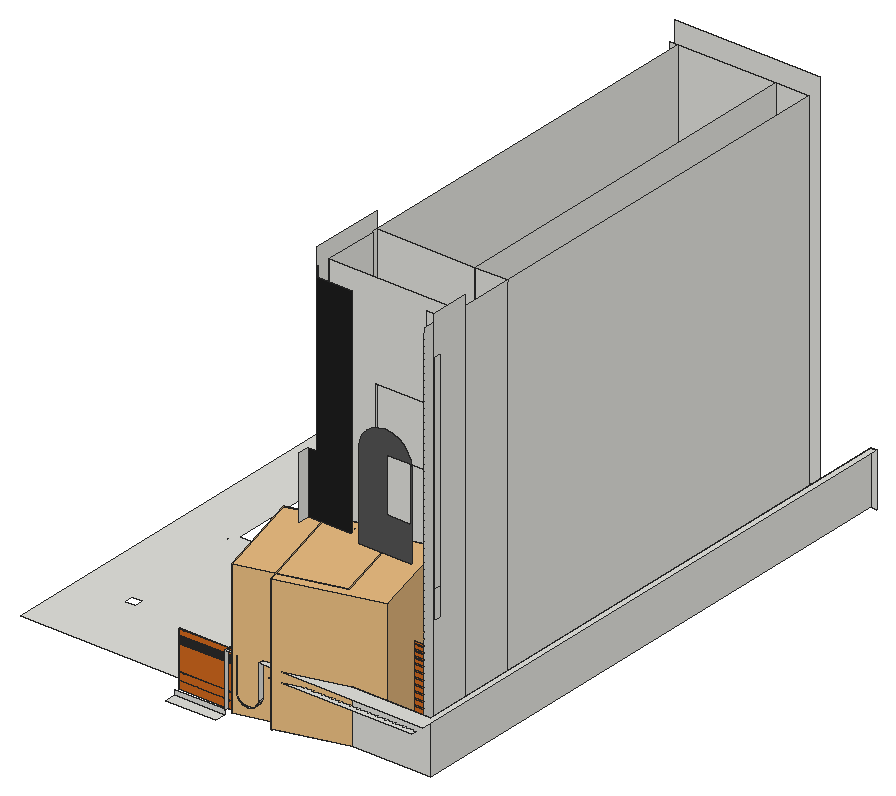
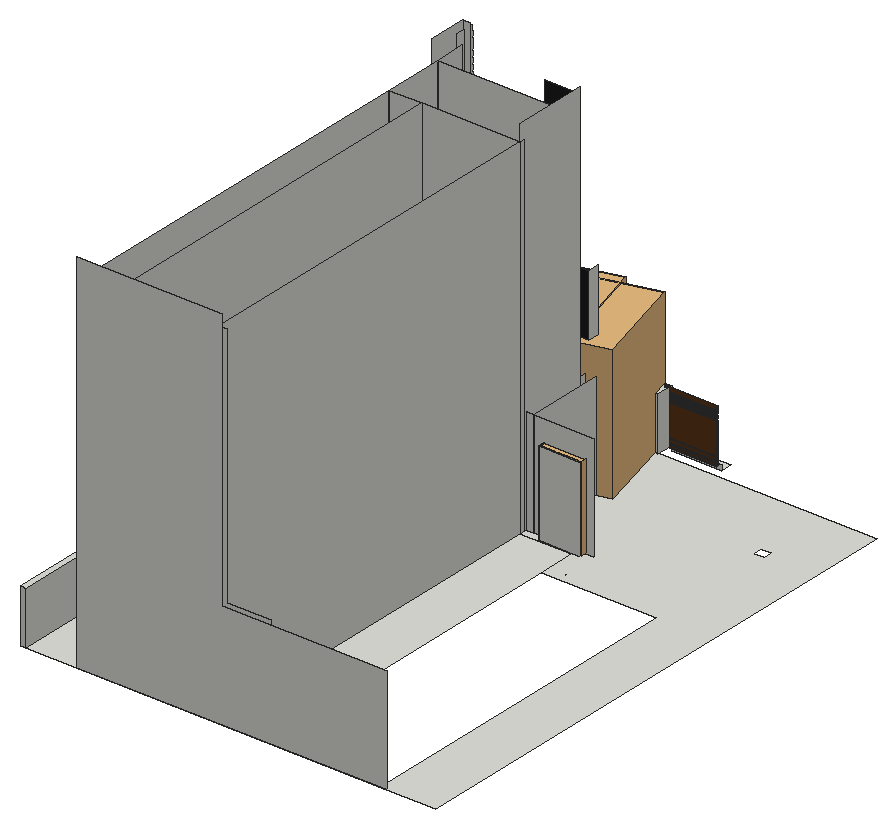
# SketchUp Ruby script. Lengths in inches.
U = 1.inch
M = Sketchup.active_model
def pt(a) = Geom::Point3d.new(a.map { |v| v * U })
def face(e, loops, mat)
  f = e.add_face(loops[0].map { |a| pt(a) })
  loops[1..].each { |l| e.add_face(l.map { |a| pt(a) }).erase! }
  f.material = f.back_material = mat if mat
  f
end
# faces: each face lists its corners as indices into pts; further lists are holes
def faces(e, pts, list, mat = nil) = list.each { |f| face(e, (f[0].is_a?(Array) ? f : [f]).map { |l| l.map { |i| pts[i] } }, mat) }
# xy, xz, yz: faces in a plane at the given z, y or x. An outline is a flat list of corners, or four numbers for a rectangle; further outlines are holes
def ring(l) = l.size == 4 ? [[l[0], l[1]], [l[2], l[1]], [l[2], l[3]], [l[0], l[3]]] : l.each_slice(2).to_a
def flat(e, list, mat, &to3) = list.each { |f| face(e, (f[0].is_a?(Array) ? f : [f]).map { |l| ring(l).map { |u, v| to3.(u, v) } }, mat) }
def xy(e, z, list, mat = nil) = flat(e, list, mat) { |x, y| [x, y, z] }
def xz(e, y, list, mat = nil) = flat(e, list, mat) { |x, z| [x, y, z] }
def yz(e, x, list, mat = nil) = flat(e, list, mat) { |y, z| [x, y, z] }
def lines(e, pts, list) = list.each { |a, b| e.add_line(pt(pts[a]), pt(pts[b])) }
# prism: a flat outline (further loops are holes) pulled along v
def prism(e, loops, v, mat = nil)
  f = face(e, loops, mat); d = Geom::Vector3d.new(v.map { |x| x * U })
  f.pushpull(f.normal.samedirection?(d) ? d.length : -d.length)
end
def box(e, o, s, mat = nil) = prism(e, [[o, [o[0] + s[0], o[1], o[2]], [o[0] + s[0], o[1] + s[1], o[2]], [o[0], o[1] + s[1], o[2]]]], [0, 0, s[2]], mat)
def at(x, y, z, deg = 0) = Geom::Transformation.translation(pt([x, y, z])) * Geom::Transformation.rotation(ORIGIN, Z_AXIS, deg.degrees)
def axes(o, x, y, z) = Geom::Transformation.new([*x, 0, *y, 0, *z, 0, *pt(o).to_a, 1])
def part(name) = M.definitions.add(name)
# library, detail: a bought-in or finely detailed component or shape, given as its bounding box
def library(name, o, s) = part(name).tap { |d| box(d.entities, o, s) }
def detail(e, o, s) = box(e.add_group.entities, o, s)
def put(e, d, t, mat = nil) = e.add_instance(d, t).tap { |i| i.material = mat if mat }
def group(e, t, mat = nil) = e.add_group.tap { |g| g.transformation = t; g.material = mat if mat }.entities
root = M.entities
M.materials.add("[0041_Chocolate]").color = [210, 105, 30]
M.materials.add("[Color M06]").color = [84, 84, 84]
M.materials.add("[Color M08]").color = [30, 30, 30]
M.materials.add("[Wood Veneer 01]2").color = [94, 55, 29]
c1 = library("元件\#5",[-4.39,0,0],[5.37,35.83,90.55])
c2 = part("Slatted screen panel")
xy(c2.entities,0,[[0,0,255.91,1.97]],"[Wood Veneer 01]2")
xy(c2.entities,16.54,[[0,1.18,255.91,1.97]],"[Wood Veneer 01]2")
xy(c2.entities,16.93,[[0,0,255.91,1.18]],"[Wood Veneer 01]2")
xy(c2.entities,17.78,[[0,0,255.91,1.18]],"[Wood Veneer 01]2")
xy(c2.entities,34.45,[[0,0,255.91,1.18]],"[Wood Veneer 01]2")
xy(c2.entities,35.07,[[0,0,255.91,1.18]],"[Wood Veneer 01]2")
xy(c2.entities,89.37,[[0,0,255.91,1.97]],"[Wood Veneer 01]2")
xy(c2.entities,92.91,[[0,0,255.91,1.97]],"[Wood Veneer 01]2")
xy(c2.entities,94.49,[[0,0,255.91,1.97]],"[Wood Veneer 01]2")
xy(c2.entities,97.64,[[0,0,255.91,1.97]],"[Wood Veneer 01]2")
xy(c2.entities,99.21,[[0,0,255.91,1.97]],"[Wood Veneer 01]2")
xy(c2.entities,102.36,[[0,0,255.91,1.97]],"[Wood Veneer 01]2")
xy(c2.entities,103.9375,[[0,0,255.91,1.97]],"[Wood Veneer 01]2")
xy(c2.entities,107.48,[[0,0,255.91,1.97]],"[Wood Veneer 01]2")
xy(c2.entities,119.29,[[0,0,255.91,1.97]],"[Wood Veneer 01]2")
xz(c2.entities,0,[[0,0,255.91,16.93],[0,17.78,255.91,34.45],[0,35.07,255.91,89.37],[0,92.91,255.91,94.49],[0,97.64,255.91,99.21],
  [0,102.36,255.91,103.9375],[0,107.48,255.91,119.29]],"[0041_Chocolate]")
xz(c2.entities,1.18,[[0,16.54,255.91,16.93],[0,16.93,255.91,17.78],[0,34.45,255.91,35.07]],"[Wood Veneer 01]2")
xz(c2.entities,1.97,[[0,0,255.91,1.57],[0,1.57,255.91,5.51],[0,5.51,255.91,7.09],[0,7.09,255.91,11.8125],[0,11.8125,255.91,16.54],
  [0,16.54,255.91,19.69],[0,19.69,255.91,89.37],[0,92.91,255.91,94.49],[0,97.64,255.91,99.21],[0,102.36,255.91,103.9375],
  [0,107.48,255.91,109.84],[0,109.84,255.91,119.29]],"[Wood Veneer 01]2")
yz(c2.entities,0,[[0,0,1.97,1.57],[0,1.57,1.97,5.51],[0,5.51,1.97,7.09],[0,7.09,1.97,11.8125],[0,11.8125,0,16.93,1.18,16.93,1.18,16.54,1.97,16.54,1.97,11.8125],
  [1.18,16.54,1.97,19.69],[0,17.78,0,34.45,1.18,34.45,1.18,35.07,0,35.07,0,89.37,1.97,89.37,1.97,19.69,1.18,19.69,1.18,17.78],[0,92.91,1.97,94.49],[0,97.64,1.97,99.21],[0,102.36,1.97,103.9375],
  [0,107.48,1.97,109.84],[0,109.84,1.97,119.29]],"[Wood Veneer 01]2")
yz(c2.entities,255.91,[[0,0,1.97,1.57],[0,1.57,1.97,5.51],[0,5.51,1.97,7.09],[0,7.09,1.97,11.8125],[0,11.8125,1.97,11.8125,1.97,16.54,1.18,16.54,1.18,16.93,0,16.93],
  [1.18,16.54,1.97,19.69],[0,17.78,1.18,17.78,1.18,19.69,1.97,19.69,1.97,89.37,0,89.37,0,35.07,1.18,35.07,1.18,34.45,0,34.45],[0,92.91,1.97,94.49],[0,97.64,1.97,99.21],[0,102.36,1.97,103.9375],
  [0,107.48,1.97,109.84],[0,109.84,1.97,119.29]],"[Wood Veneer 01]2")
p = [[255.91,1.97,103.9375],[255.91,1.97,107.48],[0,1.97,107.48],[0,1.97,103.9375],[0,1.97,92.91],[0,1.97,89.37],
  [255.91,1.97,99.21],[255.91,1.97,102.36],[255.91,1.97,89.37],[255.91,1.97,92.91],[0,1.97,97.64],[0,1.97,94.49],
  [0,1.97,102.36],[0,1.97,99.21],[255.91,1.97,94.49],[255.91,1.97,97.64],[240.94,0,5.51],[240.94,1.97,5.51]]
lines(c2.entities,p,[[0,1],[2,3],[4,5],[6,7],[8,9],[10,11],[12,13],[14,15],[16,17]])
c3 = library("Palm tree",[-4.09,-4.52,0],[193.52,193.51,258.93])
c4 = part("Palm+Tree")
put(c4.entities,c3,at(25.51,-21.81,0,15))
xy(root,0.73,[[2115.83,876.83,2172.86,889.52]])
xy(root,6.125,[[[1927.01,908.02,2389.93,908.02,2389.93,1529.04,1982.33,1529.04,1982.33,1130.875,2100.82,1130.875,2100.82,1088.75,2110.86,1088.75,2110.86,1095.9375,2158.05,1095.9375,2158.05,1088.75,2177.96,1088.75,2177.96,1097.28,2119.65,1097.28,2119.65,1139.4,1989.57,1139.4,1989.57,1521.81,2326.17,1521.81,2326.17,1027.17,2332.96,1027.17,2332.96,983.34,2332.08,983.34,2332.08,971.36,2230.65,971.36,2230.65,983.34,2230.15,983.34,2230.15,996.48,2181.03,996.48,2181.03,983.34,2169.44,983.34,2169.44,1088.75,2158.05,1088.75,2158.05,1095.9375,2110.86,1095.9375,2110.86,1088.75,2100.82,1088.75,2100.82,1130.875,1982.33,1130.875,1982.33,1529.04,1927.01,1529.04],[1982.33,985.23,1995.33,996.48]],[2230.65,971.36,2326.17,971.36,2326.17,983.34,2325.29,983.34,2325.29,992.96,2230.65,992.96],[2326.17,971.36,2332.08,983.34],[2169.44,983.34,2181.03,996.48],[2230.15,983.34,2230.65,993.35],
  [2325.29,983.34,2326.17,993.35],[2326.17,983.34,2332.96,993.35],[2230.65,992.96,2325.29,993.35],[[2230.65,993.35,2326.17,993.35,2326.17,1097.28,2177.96,1097.28,2177.96,1088.75,2169.44,1088.75,2169.44,1003.71,2190.68,1003.71,2190.68,996.48,2230.65,996.48],[2177.96,1012.23,2179.15,1088.75]],[2230.65,993.35,2230.65,996.48,2190.68,996.48,2190.68,1003.71,2179.15,1003.71,2179.15,1027.17,2326.17,1027.17,2326.17,993.35],
  [2230.65,993.35,2230.65,996.48,2190.68,996.48,2190.68,1003.71,2230.65,1003.71,2230.65,996.48,2326.17,996.48,2326.17,993.35],[2230.15,993.35,2230.65,996.48],[2326.17,993.35,2332.96,996.48],[2169.44,996.48,2181.03,1003.71],[2230.65,996.48,2230.65,1003.71,2179.15,1003.71,2179.15,1027.17,2326.17,1027.17,2326.17,996.48],
  [2181.03,996.48,2190.68,1003.71],[2326.17,996.48,2332.96,1027.17],[2169.44,1003.71,2169.44,1088.75,2177.96,1088.75,2177.96,1012.23,2179.15,1012.23,2179.15,1003.71],[2177.96,1012.23,2179.15,1088.75],[2179.15,1027.17,2326.17,1028.46],
  [2179.15,1028.46,2326.17,1028.46,2326.17,1097.28,2177.96,1097.28,2177.96,1089.96,2179.15,1089.96],[2177.96,1088.75,2179.15,1089.96],[2119.65,1097.28,2177.96,1521.81],[2177.96,1097.28,2289.17,1521.81],[2289.17,1097.28,2326.17,1521.81]])
xy(root,11.08,[[2230.65,971.36,2332.08,972.36]],"[0041_Chocolate]")
xy(root,13.1875,[[2230.65,971.36,2332.08,972.36]],"[0041_Chocolate]")
xy(root,18.14,[[2230.65,971.36,2332.08,972.36]],"[0041_Chocolate]")
xy(root,20.25,[[2230.65,971.36,2332.08,972.36]],"[0041_Chocolate]")
xy(root,25.2,[[2230.65,971.36,2332.08,972.36]],"[0041_Chocolate]")
xy(root,27.3125,[[2230.65,971.36,2332.08,972.36]],"[0041_Chocolate]")
xy(root,32.27,[[2230.65,971.36,2332.08,972.36]],"[0041_Chocolate]")
xy(root,34.375,[[2230.65,971.36,2332.08,972.36]],"[0041_Chocolate]")
xy(root,39.33,[[2230.65,971.36,2332.08,972.36]],"[0041_Chocolate]")
xy(root,41.4375,[[2230.65,971.36,2332.08,972.36]],"[0041_Chocolate]")
xy(root,46.39,[[2230.65,971.36,2332.08,972.36]],"[0041_Chocolate]")
xy(root,48.5,[[2230.65,971.36,2332.08,972.36]],"[0041_Chocolate]")
xy(root,53.45,[[2230.65,971.36,2332.08,972.36]],"[0041_Chocolate]")
xy(root,55.1875,[[2221.9375,889.52,2221.9375,894.77,2223.5625,894.77,2223.5625,895.77,2224.3125,895.77,2224.3125,894.77,2227.5625,894.77,2227.5625,895.77,2228.3125,895.77,2228.3125,894.77,2231.5625,894.77,2231.5625,895.77,2232.3125,895.77,2232.3125,894.77,2235.5625,894.77,2235.5625,895.77,2236.3125,895.77,2236.3125,894.77,2239.5625,894.77,2239.5625,895.77,2240.3125,895.77,2240.3125,894.77,2243.5625,894.77,2243.5625,895.77,2244.3125,895.77,2244.3125,894.77,2247.5625,894.77,2247.5625,895.77,2248.3125,895.77,2248.3125,894.77,2251.5625,894.77,2251.5625,895.77,2252.3125,895.77,2252.3125,894.77,2255.5625,894.77,2255.5625,895.77,2256.3125,895.77,2256.3125,894.77,2259.5625,894.77,2259.5625,895.77,2260.3125,895.77,2260.3125,894.77,2263.5625,894.77,2263.5625,895.77,2264.3125,895.77,2264.3125,894.77,2267.5625,894.77,2267.5625,895.77,2268.3125,895.77,2268.3125,894.77,2271.5625,894.77,2271.5625,895.77,2272.3125,895.77,2272.3125,894.77,2275.5625,894.77,2275.5625,895.77,2276.3125,895.77,2276.3125,894.77,2279.5625,894.77,2279.5625,895.77,2280.3125,895.77,2280.3125,894.77,2283.5625,894.77,2283.5625,895.77,2284.3125,895.77,2284.3125,894.77,2287.5625,894.77,2287.5625,895.77,2288.3125,895.77,2288.3125,894.77,2291.5625,894.77,2291.5625,895.77,2292.3125,895.77,2292.3125,894.77,2295.5625,894.77,2295.5625,895.77,2296.3125,895.77,2296.3125,894.77,2299.5625,894.77,2299.5625,895.77,2300.3125,895.77,2300.3125,894.77,2303.5625,894.77,2303.5625,895.77,2304.3125,895.77,2304.3125,894.77,2307.5625,894.77,2307.5625,895.77,2308.3125,895.77,2308.3125,894.77,2311.5625,894.77,2311.5625,895.77,2312.3125,895.77,2312.3125,894.77,2315.5625,894.77,2315.5625,895.77,2316.3125,895.77,2316.3125,894.77,2319.5625,894.77,2319.5625,895.77,2320.3125,895.77,2320.3125,894.77,2323.5625,894.77,2323.5625,895.77,2324.3125,895.77,2324.3125,894.77,2327.5625,894.77,2327.5625,895.77,2328.3125,895.77,2328.3125,894.77,2331.5625,894.77,2331.5625,895.77,2332.3125,895.77,2332.3125,894.77,2335.5625,894.77,2335.5625,895.77,2336.3125,895.77,2336.3125,894.77,2339.5625,894.77,2339.5625,895.77,2340.3125,895.77,2340.3125,894.77,2343.5625,894.77,2343.5625,895.77,2344.3125,895.77,2344.3125,894.77,2347.5625,894.77,2347.5625,895.77,2348.3125,895.77,2348.3125,894.77,2351.5625,894.77,2351.5625,895.77,2352.3125,895.77,2352.3125,894.77,2355.5625,894.77,2355.5625,895.77,2356.3125,895.77,2356.3125,894.77,2359.5625,894.77,2359.5625,895.77,2360.3125,895.77,2360.3125,894.77,2363.5625,894.77,2363.5625,895.77,2364.3125,895.77,2364.3125,894.77,2367.5625,894.77,2367.5625,895.77,2368.3125,895.77,2368.3125,894.77,2371.5625,894.77,2371.5625,895.77,2372.3125,895.77,2372.3125,894.77,2375.5625,894.77,2375.5625,895.77,2376.3125,895.77,2376.3125,894.77,2379.5625,894.77,2379.5625,895.77,2380.3125,895.77,2380.3125,894.77,2383.5625,894.77,2383.5625,889.52]])
xy(root,55.5625,[[2230.65,971.36,2332.08,972.36]],"[0041_Chocolate]")
xy(root,60.52,[[2230.65,971.36,2332.08,972.36]],"[0041_Chocolate]")
xy(root,62.625,[[2230.65,971.36,2332.08,972.36]],"[0041_Chocolate]")
xy(root,66.125,[[2173.1,889.52,2186.22,889.52,2186.22,895.77,2210.54,895.77,2210.54,889.52,2396.46,889.52,2396.46,1529.04,2389.93,1529.04,2389.93,908.02,2173.1,908.02]])
xy(root,67.58,[[2230.65,971.36,2332.08,972.36]],"[0041_Chocolate]")
xy(root,69.6875,[[2230.65,971.36,2332.08,972.36]],"[0041_Chocolate]")
xy(root,74.64,[[2230.65,971.36,2266.85,972.36],[2284.79,971.36,2332.08,972.36]],"[0041_Chocolate]")
xy(root,76.75,[[2230.65,971.36,2261.76,972.36],[2289.88,971.36,2332.08,972.36]],"[0041_Chocolate]")
xy(root,81.7,[[2230.65,971.36,2254.92,972.36],[2296.72,971.36,2332.08,972.36]],"[0041_Chocolate]")
xy(root,83.8125,[[2230.65,971.36,2253.24,972.36],[2298.41,971.36,2332.08,972.36]],"[0041_Chocolate]")
xy(root,88.77,[[2230.65,971.36,2249.71,972.36],[2301.9375,971.36,2332.08,972.36]],"[0041_Chocolate]")
xz(root,889.52,[[2115.83,0.73,2172.86,6.125]])
xz(root,895.77,[[2220.3125,0,2221.9375,55.1875]])
xz(root,895.77,[[2198.38,16.91,2201.18,17.23,2203.84,18.17,2206.21,19.69,2208.18,21.71,2209.65,24.11,2210.54,26.79,2210.54,66.125,2186.22,66.125,2186.22,26.79,2187.11,24.11,2188.58,21.71,2190.55,19.69,2192.92,18.17,2195.58,17.23]],"[0041_Chocolate]")
xz(root,908.02,[[2173.1,6.125,2389.93,66.125]])
xz(root,971.36,[[2230.65,6.125,2332.08,11.08],[2230.65,13.1875,2332.08,18.14],[2230.65,20.25,2332.08,25.2],[2230.65,27.3125,2332.08,32.27],[2230.65,34.375,2332.08,39.33],
  [2230.65,41.4375,2332.08,46.39],[2230.65,48.5,2332.08,53.45],[2230.65,55.5625,2332.08,60.52],[2230.65,62.625,2332.08,67.58],[2230.65,69.6875,2332.08,69.6875,2332.08,74.64,2284.79,74.64,2283.53,74.12,2275.82,73.1,2268.11,74.12,2266.85,74.64,2230.65,74.64],
  [2230.65,76.75,2261.76,76.75,2260.93,77.09,2254.92,81.7,2230.65,81.7],[2289.88,76.75,2332.08,76.75,2332.08,81.7,2296.72,81.7,2290.72,77.09],[2230.65,83.8125,2253.24,83.8125,2250.02,88,2249.71,88.77,2230.65,88.77],[2298.41,83.8125,2332.08,83.8125,2332.08,88.77,2301.9375,88.77,2301.62,88]],"[0041_Chocolate]")
xz(root,972.36,[[2230.65,11.08,2332.08,13.1875],[2230.65,18.14,2332.08,20.25],[2230.65,25.2,2332.08,27.3125],[2230.65,32.27,2332.08,34.375],[2230.65,39.33,2332.08,41.4375],
  [2230.65,46.39,2332.08,48.5],[2230.65,53.45,2332.08,55.5625],[2230.65,60.52,2332.08,62.625],[2230.65,67.58,2332.08,69.6875],[2230.65,74.64,2266.85,74.64,2261.76,76.75,2230.65,76.75],
  [2284.79,74.64,2332.08,74.64,2332.08,76.75,2289.88,76.75],[2230.65,81.7,2254.92,81.7,2254.76,81.83,2253.24,83.8125,2230.65,83.8125],[2296.72,81.7,2332.08,81.7,2332.08,83.8125,2298.41,83.8125,2296.88,81.83],[2230.65,88.77,2249.71,88.77,2248.83,90.875,2230.65,90.875],[2301.9375,88.77,2332.08,88.77,2332.08,90.875,2302.81,90.875]],"[0041_Chocolate]")
xz(root,983.34,[[2169.44,6.125,2181.03,132.47],[2325.29,6.125,2326.17,126.125],[2326.17,6.125,2332.08,126.125],[2332.08,6.125,2332.96,6.125,2332.96,421.25,2326.17,421.25,2326.17,141.26,2332.08,141.26]])
xz(root,986.55,[[[2275.82,73.1,2283.53,74.12,2284.79,74.64,2289.88,76.75,2290.72,77.09,2296.72,81.7,2296.88,81.83,2298.41,83.8125,2301.62,88,2301.9375,88.77,2302.81,90.875,2304.59,95.18,2304.68,95.83,2304.87,97.27,2280.42,97.27,2280.42,145.27,2305.61,145.27,2305.61,253.3125,2304.96,258.27,2304.68,260.375,2304.59,261.02,2302.81,265.33,2301.9375,267.4375,2301.62,268.21,2298.41,272.39,2296.88,274.375,2296.72,274.5,2290.72,279.11,2289.88,279.45,2284.79,281.5625,2283.53,282.09,2275.82,283.1,2268.11,282.09,2266.85,281.5625,2261.76,279.45,2260.93,279.11,2254.92,274.5,2254.76,274.375,2253.24,272.39,2250.02,268.21,2249.71,267.4375,2248.83,265.33,2247.05,261.02,2246.96,260.375,2246.69,258.27,2246.03,253.3125,2246.03,102.89,2246.69,97.9375,2246.96,95.83,2247.05,95.18,2248.83,90.875,2249.71,88.77,2250.02,88,2253.24,83.8125,2254.76,81.83,2254.92,81.7,2260.93,77.09,2261.76,76.75,2266.85,74.64,2268.11,74.12],[2278.27,196.89,2304.96,258.27]]],"[Color M06]")
xz(root,993.35,[[2230.15,6.125,2230.65,8.32],[2230.65,6.125,2317.62,8.32],[2317.62,6.125,2325.29,8.32],[2325.29,6.125,2326.17,8.32],[2326.17,6.125,2332.96,8.32],
  [2230.15,8.32,2230.65,95.62],[2230.65,8.32,2317.62,126.125],[2317.62,8.32,2325.29,109.9375],[2325.29,8.32,2326.17,109.9375]])
xz(root,996.48,[[2181.03,6.125,2230.15,6.125,2230.15,126.125,2230.65,126.125,2230.65,402.64,2190.68,402.64,2190.68,226.8,2181.03,226.8]],"[Color M08]")
xz(root,1003.71,[[2179.15,6.125,2181.03,126.125],[2181.03,6.125,2190.68,126.125]])
xz(root,1012.23,[[2177.96,6.125,2179.15,402.64]])
xz(root,1028.46,[[[2179.15,6.125,2326.17,402.64],[2230.65,226.8,2323.46,295.72]]])
xz(root,1088.75,[[2100.82,6.125,2110.86,6.125,2110.86,101.1875,2158.05,101.1875,2158.05,6.125,2169.44,6.125,2169.44,126.125,2100.82,126.125],[2169.44,6.125,2179.15,126.125]])
xz(root,1089.96,[[2177.96,6.125,2179.15,402.64]])
xz(root,1095.9375,[[2110.86,6.125,2158.05,101.1875]])
xz(root,1097.28,[[2177.96,6.125,2289.17,402.64],[2289.17,6.125,2326.17,402.64]])
xz(root,1521.81,[[2119.65,6.125,2119.65,126.125,2169.44,126.125,2169.44,402.64,2177.96,402.64,2177.96,6.125],[2177.96,6.125,2289.17,402.64],[2289.17,6.125,2326.17,402.64]])
xz(root,1529.04,[[1982.33,6.125,1982.33,126.125,2169.44,126.125,2169.44,421.25,2332.96,421.25,2332.96,6.125],[2389.93,6.125,2396.46,66.125]])
yz(root,2158.05,[[1088.75,6.125,1095.9375,101.1875]])
yz(root,2169.44,[[983.34,6.125,983.34,132.47,996.48,132.47,996.48,126.125,1088.75,126.125,1088.75,6.125]])
yz(root,2173.1,[[889.52,6.125,908.02,66.125]])
yz(root,2177.96,[[1012.23,6.125,1012.23,421.25,1097.28,421.25,1097.28,402.64,1089.96,402.64,1089.96,6.125],[1089.96,6.125,1097.28,402.64],[1097.28,6.125,1521.81,402.64]])
yz(root,2179.15,[[1003.71,6.125,1012.23,126.125],[1012.23,6.125,1027.17,126.125],[1027.17,6.125,1028.46,126.125],[1028.46,6.125,1088.75,126.125],[1088.75,6.125,1089.96,6.125,1089.96,402.64,1028.46,402.64,1028.46,126.125,1088.75,126.125]])
yz(root,2181.03,[[983.34,6.125,996.48,226.8]])
yz(root,2186.22,[[889.52,26.79,895.77,66.125]])
yz(root,2210.54,[[889.52,26.79,895.77,66.125]])
yz(root,2221.9375,[[894.77,0,895.77,55.1875]])
yz(root,2230.15,[[993.35,6.125,996.48,8.32],[993.35,8.32,996.48,95.62]])
yz(root,2230.65,[[971.36,6.125,971.36,11.08,972.36,11.08,972.36,13.1875,971.36,13.1875,971.36,18.14,972.36,18.14,972.36,20.25,971.36,20.25,971.36,25.2,972.36,25.2,972.36,27.3125,971.36,27.3125,971.36,32.27,972.36,32.27,972.36,34.375,971.36,34.375,971.36,39.33,972.36,39.33,972.36,41.4375,971.36,41.4375,971.36,46.39,972.36,46.39,972.36,48.5,971.36,48.5,971.36,53.45,972.36,53.45,972.36,55.5625,971.36,55.5625,971.36,60.52,972.36,60.52,972.36,62.625,971.36,62.625,971.36,67.58,972.36,67.58,972.36,69.6875,971.36,69.6875,971.36,74.64,972.36,74.64,972.36,76.75,971.36,76.75,971.36,81.7,972.36,81.7,972.36,83.8125,971.36,83.8125,971.36,88.77,972.36,88.77,972.36,90.875,971.36,90.875,971.36,95.83,972.36,95.83,972.36,97.9375,971.36,97.9375,971.36,102.89,972.36,102.89,972.36,105,971.36,105,971.36,109.95,972.36,109.95,972.36,112.0625,971.36,112.0625,971.36,117.02,972.36,117.02,972.36,119.125,971.36,119.125,971.36,124.08,972.36,124.08,972.36,126.1875,971.36,126.1875,971.36,131.14,972.36,131.14,972.36,133.25,971.36,133.25,971.36,138.2,972.36,138.2,972.36,140.3125,971.36,140.3125,971.36,141.26,983.34,141.26,983.34,126.125,993.35,126.125,993.35,6.125]])
yz(root,2289.17,[[1097.28,6.125,1521.81,402.64]])
yz(root,2325.29,[[983.34,6.125,993.35,126.125]])
yz(root,2326.17,[[993.35,6.125,1028.46,402.64],[1028.46,6.125,1097.28,402.64],[1097.28,6.125,1521.81,402.64]])
yz(root,2332.08,[[971.36,6.125,983.34,6.125,983.34,141.26,993.35,141.26,993.35,411.82,972.36,411.82,972.36,405.64,971.36,405.64,971.36,400.6875,972.36,400.6875,972.36,398.77,971.36,398.77,971.36,393.8125,972.36,393.8125,972.36,391.89,971.36,391.89,971.36,386.9375,972.36,386.9375,972.36,385.02,971.36,385.02,971.36,380.0625,972.36,380.0625,972.36,378.14,971.36,378.14,971.36,373.1875,972.36,373.1875,972.36,371.27,971.36,371.27,971.36,366.3125,972.36,366.3125,972.36,364.2,971.36,364.2,971.36,359.25,972.36,359.25,972.36,357.14,971.36,357.14,971.36,352.1875,972.36,352.1875,972.36,350.08,971.36,350.08,971.36,345.125,972.36,345.125,972.36,343.02,971.36,343.02,971.36,338.0625,972.36,338.0625,972.36,335.95,971.36,335.95,971.36,331,972.36,331,972.36,328.89,971.36,328.89,971.36,323.9375,972.36,323.9375,972.36,321.83,971.36,321.83,971.36,316.875,972.36,316.875,972.36,314.77,971.36,314.77,971.36,309.8125,972.36,309.8125,972.36,307.7,971.36,307.7,971.36,302.75,972.36,302.75,972.36,300.64,971.36,300.64,971.36,295.6875,972.36,295.6875,972.36,293.58,971.36,293.58,971.36,288.625,972.36,288.625,972.36,286.52,971.36,286.52,971.36,281.5625,972.36,281.5625,972.36,279.45,971.36,279.45,971.36,274.5,972.36,274.5,972.36,272.39,971.36,272.39,971.36,267.4375,972.36,267.4375,972.36,265.33,971.36,265.33,971.36,260.375,972.36,260.375,972.36,258.27,971.36,258.27,971.36,253.3125,972.36,253.3125,972.36,251.2,971.36,251.2,971.36,246.25,972.36,246.25,972.36,244.14,971.36,244.14,971.36,239.1875,972.36,239.1875,972.36,237.08,971.36,237.08,971.36,232.125,972.36,232.125,972.36,230.02,971.36,230.02,971.36,225.0625,972.36,225.0625,972.36,222.95,971.36,222.95,971.36,218,972.36,218,972.36,215.89,971.36,215.89,971.36,210.9375,972.36,210.9375,972.36,208.83,971.36,208.83,971.36,203.875,972.36,203.875,972.36,201.77,971.36,201.77,971.36,196.8125,972.36,196.8125,972.36,194.7,971.36,194.7,971.36,189.75,972.36,189.75,972.36,187.64,971.36,187.64,971.36,182.6875,972.36,182.6875,972.36,180.58,971.36,180.58,971.36,175.625,972.36,175.625,972.36,173.52,971.36,173.52,971.36,168.5625,972.36,168.5625,972.36,166.45,971.36,166.45,971.36,161.5,972.36,161.5,972.36,159.39,971.36,159.39,971.36,154.4375,972.36,154.4375,972.36,152.33,971.36,152.33,971.36,147.375,972.36,147.375,972.36,145.27,971.36,145.27,971.36,140.3125,972.36,140.3125,972.36,138.2,971.36,138.2,971.36,133.25,972.36,133.25,972.36,131.14,971.36,131.14,971.36,126.1875,972.36,126.1875,972.36,124.08,971.36,124.08,971.36,119.125,972.36,119.125,972.36,117.02,971.36,117.02,971.36,112.0625,972.36,112.0625,972.36,109.95,971.36,109.95,971.36,105,972.36,105,972.36,102.89,971.36,102.89,971.36,97.9375,972.36,97.9375,972.36,95.83,971.36,95.83,971.36,90.875,972.36,90.875,972.36,88.77,971.36,88.77,971.36,83.8125,972.36,83.8125,972.36,81.7,971.36,81.7,971.36,76.75,972.36,76.75,972.36,74.64,971.36,74.64,971.36,69.6875,972.36,69.6875,972.36,67.58,971.36,67.58,971.36,62.625,972.36,62.625,972.36,60.52,971.36,60.52,971.36,55.5625,972.36,55.5625,972.36,53.45,971.36,53.45,971.36,48.5,972.36,48.5,972.36,46.39,971.36,46.39,971.36,41.4375,972.36,41.4375,972.36,39.33,971.36,39.33,971.36,34.375,972.36,34.375,972.36,32.27,971.36,32.27,971.36,27.3125,972.36,27.3125,972.36,25.2,971.36,25.2,971.36,20.25,972.36,20.25,972.36,18.14,971.36,18.14,971.36,13.1875,972.36,13.1875,972.36,11.08,971.36,11.08]])
yz(root,2332.96,[[983.34,6.125,1027.17,6.125,1027.17,421.25,983.34,421.25,983.34,376.875,993.35,376.875,993.35,109.9375,990,109.9375,985.91,110.21,983.34,110.72]])
yz(root,2389.93,[[908.02,6.125,1529.04,66.125]])
p = [[2198.38,895.77,16.91],[2195.58,895.77,17.23],[2195.58,889.52,17.23],[2198.38,889.52,16.91],[2201.18,895.77,17.23],[2201.18,889.52,17.23],
  [2192.92,895.77,18.17],[2192.92,889.52,18.17],[2203.84,895.77,18.17],[2203.84,889.52,18.17],[2190.55,895.77,19.69],[2190.55,889.52,19.69],
  [2206.21,895.77,19.69],[2206.21,889.52,19.69],[2188.58,895.77,21.71],[2188.58,889.52,21.71],[2208.18,895.77,21.71],[2208.18,889.52,21.71],
  [2187.11,895.77,24.11],[2187.11,889.52,24.11],[2209.65,895.77,24.11],[2209.65,889.52,24.11],[2186.22,895.77,26.79],[2186.22,889.52,26.79],
  [2210.54,895.77,26.79],[2210.54,889.52,26.79],[2268.11,986.55,74.12],[2268.11,971.36,74.12],[2275.82,971.36,73.1],[2275.82,986.55,73.1],
  [2283.53,971.36,74.12],[2283.53,986.55,74.12],[2266.85,986.55,74.64],[2266.85,972.36,74.64],[2266.85,971.36,74.64],[2284.79,971.36,74.64],
  [2284.79,972.36,74.64],[2284.79,986.55,74.64],[2261.76,972.36,76.75],[2261.76,986.55,76.75],[2289.88,972.36,76.75],[2289.88,986.55,76.75],
  [2260.93,986.55,77.09],[2260.93,971.36,77.09],[2261.76,971.36,76.75],[2289.88,971.36,76.75],[2290.72,971.36,77.09],[2290.72,986.55,77.09],
  [2254.92,986.55,81.7],[2254.92,972.36,81.7],[2254.92,971.36,81.7],[2296.72,971.36,81.7],[2296.72,972.36,81.7],[2296.72,986.55,81.7],
  [2254.76,972.36,81.83],[2254.76,986.55,81.83],[2296.88,972.36,81.83],[2296.88,986.55,81.83],[2253.24,972.36,83.8125],[2253.24,986.55,83.8125],
  [2298.41,972.36,83.8125],[2298.41,986.55,83.8125],[2250.02,986.55,88],[2250.02,971.36,88],[2253.24,971.36,83.8125],[2298.41,971.36,83.8125],
  [2301.62,971.36,88],[2301.62,986.55,88],[2249.71,986.55,88.77],[2249.71,972.36,88.77],[2249.71,971.36,88.77],[2301.9375,971.36,88.77],
  [2301.9375,972.36,88.77],[2301.9375,986.55,88.77],[2248.83,972.36,90.875],[2248.83,986.55,90.875],[2302.81,972.36,90.875],[2302.81,986.55,90.875],
  [2230.65,1003.71,24.125],[2230.65,1003.71,6.125],[2230.65,1012.23,24.125]]
faces(root,p,[[0,1,2,3],[4,0,3,5],[1,6,7,2],[8,4,5,9],[6,10,11,7],[12,8,9,13],[10,14,15,11],[16,12,13,17],
  [14,18,19,15],[20,16,17,21],[18,22,23,19],[24,20,21,25]])
faces(root,p,[[26,27,28,29],[29,28,30,31],[32,33,34,27,26],[31,30,35,36,37],[38,33,32,39],[36,40,41,37],[42,43,44,38,39],[41,40,45,46,47],
  [48,49,50,43,42],[47,46,51,52,53],[54,49,48,55],[52,56,57,53],[58,54,55,59],[56,60,61,57],[62,63,64,58,59],[61,60,65,66,67],
  [68,69,70,63,62],[67,66,71,72,73],[74,69,68,75],[72,76,77,73]],"[Color M06]")
lines(root,p,[[78,79],[78,80]])
put(root,c1,axes([2110.86,1089.14,6.11],[0,-1.05,0],[1.302,0,0],[0,0,1.05]))
put(root,c2,axes([2117.93,892.77,6.125],[0.23355,0,0],[0,0.5124,0],[0,0,0.5124]),"[0041_Chocolate]")
put(root,c4,axes([2168.73,903.83,6.125],[0.58344,0,0],[0,0.58344,0],[0,0,0.58344]),"[Color M06]")
put(root,c4,axes([2212.54,903.83,6.125],[0.58344,0,0],[0,0.58344,0],[0,0,0.58344]),"[Color M06]")
